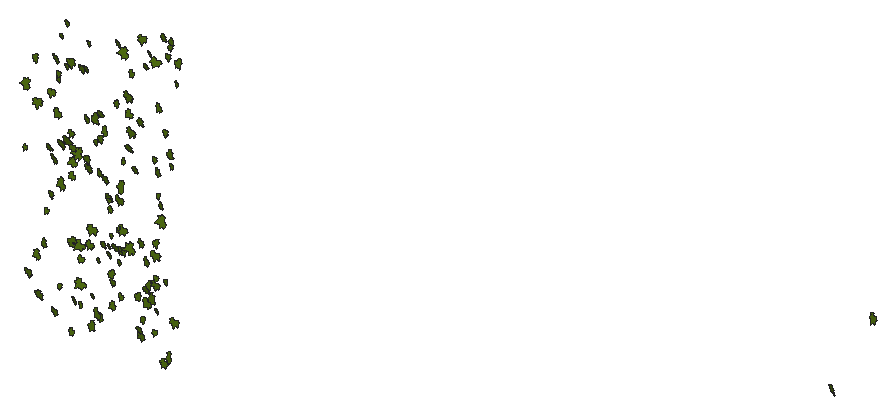
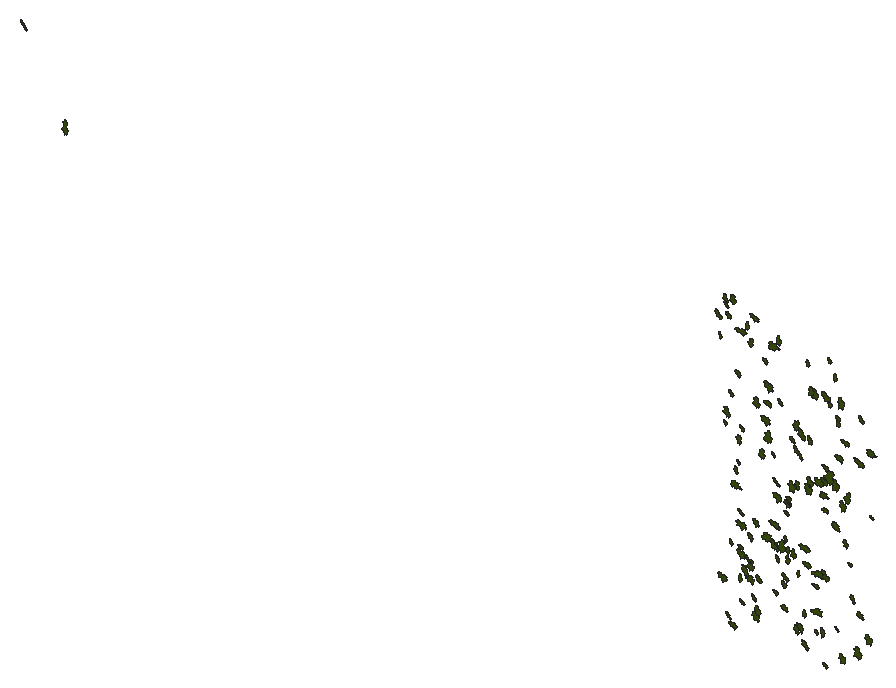
# SketchUp Ruby script. Lengths in inches.
U = 1.inch
M = Sketchup.active_model
def pt(a) = Geom::Point3d.new(a.map { |v| v * U })
def face(e, loops, mat)
  f = e.add_face(loops[0].map { |a| pt(a) })
  loops[1..].each { |l| e.add_face(l.map { |a| pt(a) }).erase! }
  f.material = f.back_material = mat if mat
  f
end
# faces: each face lists its corners as indices into pts; further lists are holes
def faces(e, pts, list, mat = nil) = list.each { |f| face(e, (f[0].is_a?(Array) ? f : [f]).map { |l| l.map { |i| pts[i] } }, mat) }
# xy, xz, yz: faces in a plane at the given z, y or x. An outline is a flat list of corners, or four numbers for a rectangle; further outlines are holes
def ring(l) = l.size == 4 ? [[l[0], l[1]], [l[2], l[1]], [l[2], l[3]], [l[0], l[3]]] : l.each_slice(2).to_a
def flat(e, list, mat, &to3) = list.each { |f| face(e, (f[0].is_a?(Array) ? f : [f]).map { |l| ring(l).map { |u, v| to3.(u, v) } }, mat) }
def xy(e, z, list, mat = nil) = flat(e, list, mat) { |x, y| [x, y, z] }
def xz(e, y, list, mat = nil) = flat(e, list, mat) { |x, z| [x, y, z] }
def yz(e, x, list, mat = nil) = flat(e, list, mat) { |y, z| [x, y, z] }
def lines(e, pts, list) = list.each { |a, b| e.add_line(pt(pts[a]), pt(pts[b])) }
# prism: a flat outline (further loops are holes) pulled along v
def prism(e, loops, v, mat = nil)
  f = face(e, loops, mat); d = Geom::Vector3d.new(v.map { |x| x * U })
  f.pushpull(f.normal.samedirection?(d) ? d.length : -d.length)
end
def box(e, o, s, mat = nil) = prism(e, [[o, [o[0] + s[0], o[1], o[2]], [o[0] + s[0], o[1] + s[1], o[2]], [o[0], o[1] + s[1], o[2]]]], [0, 0, s[2]], mat)
def at(x, y, z, deg = 0) = Geom::Transformation.translation(pt([x, y, z])) * Geom::Transformation.rotation(ORIGIN, Z_AXIS, deg.degrees)
def axes(o, x, y, z) = Geom::Transformation.new([*x, 0, *y, 0, *z, 0, *pt(o).to_a, 1])
def part(name) = M.definitions.add(name)
# library, detail: a bought-in or finely detailed component or shape, given as its bounding box
def library(name, o, s) = part(name).tap { |d| box(d.entities, o, s) }
def detail(e, o, s) = box(e.add_group.entities, o, s)
def put(e, d, t, mat = nil) = e.add_instance(d, t).tap { |i| i.material = mat if mat }
def group(e, t, mat = nil) = e.add_group.tap { |g| g.transformation = t; g.material = mat if mat }.entities
root = M.entities
M.materials.add("[Vegetation Blur 03]").color = [83, 114, 18]
c1 = part("ivy")
xy(c1.entities,0,[[0.782,0,0.786,0,0.787,0.005,0.789,0.009,0.821,0.072,0.875,0.147,1.001,0.272,1.073,0.331,1.137,0.363,1.178,0.379,1.223,0.384,1.272,0.383,1.311,0.374,1.36,0.355,1.399,0.334,1.491,0.285,1.541,0.244,1.583,0.199,1.617,0.15,1.64,0.128,1.662,0.115,1.717,0.105,1.745,0.093,1.784,0.054,1.819,0.057,1.854,0.064,1.882,0.075,1.896,0.074,1.91,0.071,1.937,0.063,1.964,0.053,1.99,0.038,2.016,0.015,2.034,0.002,2.04,0,2.038,0.003,2.036,0.007,2.033,0.038,2.036,0.068,2.045,0.1,2.055,0.116,2.064,0.123,2.077,0.129,2.088,0.129,2.106,0.132,2.118,0.13,2.179,0.132,2.207,0.133,2.225,0.133,2.242,0.138,2.22,0.162,2.207,0.186,2.206,0.213,2.212,0.236,2.228,0.262,2.247,0.274,2.298,0.283,2.355,0.294,2.37,0.296,2.376,0.295,2.377,0.3,2.377,0.303,2.385,0.329,2.411,0.37,2.426,0.392,2.449,0.407,2.511,0.426,2.561,0.444,2.619,0.466,2.589,0.469,2.561,0.476,2.501,0.5,2.449,0.516,2.424,0.523,2.401,0.535,2.377,0.556,2.372,0.568,2.36,0.575,2.268,0.586,2.225,0.592,2.207,0.599,2.194,0.61,2.143,0.65,2.13,0.664,2.122,0.682,2.123,0.7,2.13,0.719,2.148,0.75,2.17,0.781,2.195,0.807,2.221,0.828,2.284,0.874,2.291,0.88,2.288,0.887,2.276,0.9,2.267,0.916,2.265,0.933,2.273,0.967,2.292,1.002,2.313,1.03,2.334,1.054,2.348,1.067,2.358,1.074,2.363,1.076,2.362,1.081,2.35,1.094,2.347,1.11,2.35,1.143,2.359,1.18,2.385,1.254,2.415,1.324,2.448,1.393,2.45,1.4,2.446,1.398,2.44,1.394,2.427,1.383,2.402,1.36,2.376,1.339,2.345,1.324,2.305,1.309,2.282,1.303,2.273,1.306,2.245,1.294,2.212,1.287,2.187,1.291,2.163,1.301,2.142,1.316,2.134,1.327,2.124,1.325,2.09,1.292,2.053,1.259,2.014,1.234,1.973,1.215,1.954,1.21,1.931,1.208,1.909,1.212,1.893,1.22,1.879,1.233,1.872,1.248,1.867,1.281,1.864,1.319,1.821,1.258,1.773,1.197,1.726,1.141,1.698,1.121,1.679,1.116,1.666,1.117,1.647,1.122,1.632,1.129,1.62,1.141,1.617,1.154,1.617,1.219,1.621,1.254,1.623,1.268,1.623,1.281,1.618,1.314,1.606,1.346,1.603,1.375,1.607,1.403,1.603,1.467,1.599,1.499,1.605,1.525,1.614,1.552,1.629,1.577,1.635,1.589,1.629,1.587,1.618,1.582,1.596,1.566,1.581,1.556,1.568,1.552,1.557,1.55,1.545,1.553,1.531,1.562,1.522,1.572,1.504,1.591,1.486,1.611,1.474,1.631,1.457,1.666,1.455,1.684,1.457,1.698,1.452,1.715,1.444,1.728,1.424,1.754,1.419,1.772,1.423,1.786,1.434,1.819,1.444,1.848,1.446,1.855,1.44,1.861,1.43,1.867,1.386,1.904,1.349,1.948,1.326,1.973,1.31,1.995,1.288,2.048,1.284,2.153,1.287,2.254,1.284,2.255,1.282,2.253,1.278,2.247,1.274,2.237,1.266,2.216,1.226,2.125,1.208,2.076,1.184,2.033,1.155,1.984,1.135,1.942,1.111,1.899,1.083,1.861,1.053,1.85,1.059,1.83,1.061,1.809,1.056,1.79,1.049,1.767,1.04,1.749,1.018,1.733,0.994,1.726,0.942,1.734,0.95,1.6875,0.944,1.645,0.932,1.608,0.911,1.585,0.881,1.58,0.854,1.582,0.828,1.588,0.785,1.618,0.773,1.625,0.775,1.614,0.779,1.598,0.796,1.502,0.818,1.402,0.861,1.283,0.882,1.224,0.894,1.174,0.892,1.148,0.886,1.123,0.881,1.107,0.872,1.099,0.849,1.094,0.818,1.092,0.789,1.098,0.762,1.107,0.753,1.113,0.721,1.139,0.698,1.163,0.678,1.194,0.665,1.224,0.628,1.28,0.612,1.312,0.606,1.327,0.606,1.314,0.599,1.282,0.594,1.267,0.581,1.256,0.544,1.245,0.512,1.244,0.473,1.249,0.444,1.256,0.382,1.288,0.339,1.306,0.324,1.316,0.317,1.324,0.309,1.326,0.27,1.314,0.227,1.313,0.185,1.3125,0.152,1.317,0.122,1.328,0.092,1.345,0.073,1.353,0.079,1.338,0.092,1.308,0.117,1.249,0.13,1.215,0.139,1.164,0.147,1.148,0.157,1.136,0.163,1.122,0.174,1.086,0.177,1.067,0.182,1.054,0.186,1.043,0.191,1.038,0.211,1.028,0.237,1.005,0.25,0.974,0.253,0.96,0.25,0.944,0.242,0.914,0.243,0.906,0.249,0.902,0.26,0.894,0.289,0.88,0.307,0.873,0.322,0.862,0.364,0.799,0.403,0.738,0.431,0.709,0.439,0.691,0.441,0.678,0.4375,0.66,0.428,0.645,0.394,0.623,0.303,0.594,0.255,0.581,0.214,0.577,0.179,0.573,0.173,0.568,0.175,0.561,0.167,0.55,0.141,0.523,0.113,0.503,0.077,0.49,0.045,0.486,0.026,0.485,0.019,0.486,0.011,0.483,0,0.471,0.014,0.467,0.044,0.455,0.058,0.447,0.07,0.438,0.097,0.411,0.125,0.394,0.158,0.377,0.174,0.366,0.182,0.359,0.185,0.361,0.242,0.331,0.253,0.316,0.258,0.303,0.262,0.283,0.274,0.278,0.308,0.274,0.341,0.252,0.366,0.226,0.366,0.222,0.37,0.22,0.38,0.221,0.395,0.221,0.425,0.216,0.45,0.207,0.465,0.192,0.473,0.178,0.484,0.15,0.489,0.116,0.483,0.089,0.468,0.058,0.45,0.035,0.435,0.018,0.429,0.011,0.434,0.012,0.438,0.014,0.469,0.019,0.542,0.016,0.581,0.015,0.612,0.027,0.68,0.055,0.696,0.057,0.712,0.052,0.73,0.045,0.741,0.036,0.766,0.014]])
put(root,c1,axes([24.02,173.2,118.26],[0.59751,-0.1415,-0.08723],[-0.11552,-0.16395,-0.48523],[-0.05298,-1.23827,0.07421]),"[Vegetation Blur 03]")
put(root,c1,axes([30.52,173.2,121.6875],[0.30037,-0.23448,-0.48095],[-0.59958,-0.05449,-0.24524],[-0.02777,-1.36002,0.09275]),"[Vegetation Blur 03]")
put(root,c1,axes([14.2,173.2,137.15],[0.5598,-0.34639,0.09978],[0.13771,0.07562,-0.47332],[-0.15594,-1.17668,-0.05979]),"[Vegetation Blur 03]")
put(root,c1,axes([11.29,173.2,135.72],[0.34108,-0.07651,0.26436],[0.30846,-0.23678,-0.27587],[-0.10562,-0.93855,0.04805]),"[Vegetation Blur 03]")
put(root,c1,axes([32.13,173.2,139.74],[0.30667,-0.21087,0.08542],[0.09735,-0.07998,-0.26385],[-0.10945,-0.662,0.00467]),"[Vegetation Blur 03]")
put(root,c1,axes([22.87,173.2,114.92],[0.32867,-0.28906,0.36046],[0.45664,0.0115,-0.27589],[-0.07923,-1.13284,-0.09478]),"[Vegetation Blur 03]")
put(root,c1,axes([31.43,173.2,104.15],[0.33567,-0.36714,-0.32626],[-0.40941,0.10373,-0.29893],[-0.15499,-1.06915,0.08303]),"[Vegetation Blur 03]")
put(root,c1,axes([23.38,173.2,142.01],[0.40968,-0.27629,0.16507],[0.21084,0.00024,-0.34848],[-0.12034,-0.94019,-0.0486]),"[Vegetation Blur 03]")
put(root,c1,axes([13.45,173.2,124.49],[0.13916,-0.21976,0.37305],[0.46529,-0.06512,-0.12164],[-0.06205,-0.98109,-0.07549]),"[Vegetation Blur 03]")
put(root,c1,axes([30.39,173.2,132.73],[0.36627,-0.13941,0.12421],[0.13945,-0.15724,-0.30166],[-0.09113,-0.8009,0.0376]),"[Vegetation Blur 03]")
put(root,c1,axes([16.95,173.2,102.27],[0.36884,-0.18268,-0.08765],[-0.12074,-0.10682,-0.30338],[-0.06956,-0.78327,0.06182]),"[Vegetation Blur 03]")
put(root,c1,axes([15.09,173.2,107.24],[0.27201,-0.08351,0.1346],[0.14493,-0.22002,-0.21655],[-0.08857,-0.61651,0.05905]),"[Vegetation Blur 03]")
put(root,c1,axes([27.82,173.2,111.51],[0.22572,0.02556,0.3673],[0.42622,-0.34586,-0.17068],[-0.14503,-0.97663,0.07006]),"[Vegetation Blur 03]")
put(root,c1,axes([11.59,173.2,105.01],[0.44693,-0.21309,0.34937],[0.42945,-0.06761,-0.37241],[-0.09772,-1.27172,-0.03874]),"[Vegetation Blur 03]")
put(root,c1,axes([29.58,173.2,136.08],[0.46163,-0.2581,-0.13642],[-0.17424,-0.01487,-0.3883],[-0.11538,-1.01019,0.04057]),"[Vegetation Blur 03]")
put(root,c1,axes([29.79,173.2,122.5625],[0.11578,-0.07742,0.31422],[0.36947,-0.22297,-0.09932],[-0.11465,-0.79672,-0.00274]),"[Vegetation Blur 03]")
put(root,c1,axes([20.81,173.2,128.5],[0.35673,-0.12377,0.22075],[0.25958,-0.16822,-0.29423],[-0.09696,-0.90576,0.02448]),"[Vegetation Blur 03]")
put(root,c1,axes([11.39,173.2,130.33],[0.60257,-0.08021,0.1387],[0.16152,-0.21723,-0.48713],[-0.06569,-1.26991,0.07457]),"[Vegetation Blur 03]")
put(root,c1,axes([21.97,173.2,120.94],[0.20255,-0.18759,0.41357],[0.50926,-0.09194,-0.17269],[-0.07578,-1.11921,-0.05513]),"[Vegetation Blur 03]")
put(root,c1,axes([16.01,173.2,126.02],[0.0827,-0.23642,0.52033],[0.64705,-0.03418,-0.07095],[-0.03151,-1.3225,-0.09118]),"[Vegetation Blur 03]")
put(root,c1,axes([24.58,173.2,127.12],[0.30532,-0.22387,-0.07925],[-0.10993,-0.04866,-0.26046],[-0.09582,-0.65751,0.04626]),"[Vegetation Blur 03]")
put(root,c1,axes([23.22,173.2,133.91],[0.28926,-0.09005,0.2261],[0.2622,-0.20395,-0.23621],[-0.09958,-0.79857,0.03483]),"[Vegetation Blur 03]")
put(root,c1,axes([22.54,173.2,120.12],[0.34373,-0.18323,-0.04475],[-0.06771,-0.09451,-0.28552],[-0.07969,-0.71,0.04955]),"[Vegetation Blur 03]")
put(root,c1,axes([13.64,173.2,118.84],[0.37427,-0.16845,0.18276],[0.21743,-0.11081,-0.31265],[-0.09784,-0.89065,0.00433]),"[Vegetation Blur 03]")
put(root,c1,axes([27.43,173.2,110.87],[0.2552,-0.21443,0.36363],[0.45118,-0.05704,-0.2162],[-0.07626,-1.05507,-0.06222]),"[Vegetation Blur 03]")
put(root,c1,axes([23.73,173.2,113.51],[0.3306,-0.20851,0.08999],[0.10594,-0.063,-0.2822],[-0.10584,-0.71438,-0.00138]),"[Vegetation Blur 03]")
put(root,c1,axes([18.64,173.2,126.18],[0.08303,-0.1967,-0.5076],[-0.62878,-0.07669,-0.06383],[0.02474,-1.28895,0.08126]),"[Vegetation Blur 03]")
put(root,c1,axes([18.94,173.2,130.79],[0.45964,-0.254,0.03008],[0.03689,-0.00973,-0.3884],[-0.12342,-0.94883,-0.00407]),"[Vegetation Blur 03]")
put(root,c1,axes([20.56,173.2,106.22],[0.52518,-0.29878,-0.23016],[-0.2856,0.04291,-0.44284],[-0.13799,-1.22592,0.0406]),"[Vegetation Blur 03]")
put(root,c1,axes([16.22,173.2,137.1],[0.56013,-0.13091,0.22183],[0.26451,-0.15182,-0.45897],[-0.08921,-1.27215,0.03195]),"[Vegetation Blur 03]")
put(root,c1,axes([30.02,173.2,144.75],[0.24867,-0.15858,0.33537],[0.40835,-0.11898,-0.21053],[-0.08971,-0.98119,-0.02867]),"[Vegetation Blur 03]")
put(root,c1,axes([22.29,173.2,114.86],[0.1642,-0.18374,0.20113],[0.24769,-0.08699,-0.14719],[-0.08574,-0.60314,-0.04004]),"[Vegetation Blur 03]")
put(root,c1,axes([28.11,173.2,142.38],[0.3403,-0.29163,0.09942],[0.13762,0.03874,-0.29588],[-0.12643,-0.74278,-0.05447]),"[Vegetation Blur 03]")
put(root,c1,axes([27.04,173.2,107.01],[0.30019,-0.07683,0.21744],[0.25164,-0.21034,-0.24309],[-0.09515,-0.7987,0.0431]),"[Vegetation Blur 03]")
put(root,c1,axes([17.96,173.2,136.88],[0.47833,-0.24749,0.17674],[0.22101,-0.01127,-0.40089],[-0.11188,-1.08043,-0.0363]),"[Vegetation Blur 03]")
put(root,c1,axes([30.26,173.2,102.99],[0.48428,-0.17048,-0.13656],[-0.17611,-0.0992,-0.39652],[-0.06201,-1.04969,0.05965]),"[Vegetation Blur 03]")
put(root,c1,axes([28.81,173.2,128.67],[0.3385,-0.12078,0.12895],[0.14584,-0.15588,-0.27795],[-0.08451,-0.75275,0.03687]),"[Vegetation Blur 03]")
put(root,c1,axes([19.52,173.2,116.72],[0.62885,-0.10059,-0.07918],[-0.103,-0.17922,-0.50906],[-0.03454,-1.29703,0.07648]),"[Vegetation Blur 03]")
put(root,c1,axes([24,173.2,114.98],[0.40007,-0.13518,0.27607],[0.33165,-0.13835,-0.33079],[-0.0935,-1.06919,0.0079]),"[Vegetation Blur 03]")
put(root,c1,axes([23.77,173.2,114.53],[0.13511,-0.04438,0.35866],[0.42367,-0.24214,-0.11102],[-0.11873,-0.91459,0.01199]),"[Vegetation Blur 03]")
put(root,c1,axes([25.83,173.2,126.07],[0.25746,-0.20708,0.31713],[0.39391,-0.05224,-0.21837],[-0.07715,-0.95777,-0.05666]),"[Vegetation Blur 03]")
put(root,c1,axes([14.8,173.2,130.3],[0.50454,-0.20666,-0.19788],[-0.2502,-0.0525,-0.4163],[-0.0792,-1.15072,0.05453]),"[Vegetation Blur 03]")
put(root,c1,axes([26.52,173.2,132.5],[0.30631,-0.15054,0.36025],[0.43855,-0.11732,-0.25607],[-0.08874,-1.09937,-0.022]),"[Vegetation Blur 03]")
put(root,c1,axes([26.79,173.2,143.9375],[0.54024,-0.08088,0.09089],[0.10321,-0.19815,-0.43637],[-0.05739,-1.11765,0.07079]),"[Vegetation Blur 03]")
put(root,c1,axes([14.9,173.2,126.11],[0.57292,-0.29787,0.17247],[0.22282,0.05394,-0.47834],[-0.12636,-1.25544,-0.06147]),"[Vegetation Blur 03]")
put(root,c1,axes([28.14,173.2,109.62],[0.16056,0.04012,0.53459],[0.63688,-0.33645,-0.12344],[-0.15436,-1.34643,0.04677]),"[Vegetation Blur 03]")
put(root,c1,axes([26.81,173.2,117.41],[0.49502,-0.2424,-0.04719],[-0.06027,-0.00753,-0.41504],[-0.11656,-1.02555,0.0142]),"[Vegetation Blur 03]")
put(root,c1,axes([24.73,173.2,135.95],[0.66254,-0.24066,-0.04091],[-0.05165,-0.00895,-0.54898],[-0.11628,-1.36725,0.01079]),"[Vegetation Blur 03]")
put(root,c1,axes([22.05,173.2,121.33],[0.43109,-0.16307,0.09857],[0.11374,-0.09903,-0.3571],[-0.08905,-0.91592,0.02106]),"[Vegetation Blur 03]")
put(root,c1,axes([31.18,173.2,144.58],[0.22749,-0.09368,0.31124],[0.37139,-0.17878,-0.18927],[-0.09787,-0.89612,0.00522]),"[Vegetation Blur 03]")
put(root,c1,axes([19.43,173.2,114.61],[0.48596,-0.138,-0.11802],[-0.15256,-0.12597,-0.39525],[-0.04619,-1.03571,0.0638]),"[Vegetation Blur 03]")
put(root,c1,axes([25.83,173.2,116.5],[0.32603,-0.13943,-0.47145],[-0.58131,-0.12239,-0.26207],[0.01889,-1.35947,0.07195]),"[Vegetation Blur 03]")
put(root,c1,axes([29.16,173.2,108.93],[0.26661,-0.22568,0.1584],[0.20153,-0.02212,-0.2309],[-0.09528,-0.67823,-0.04518]),"[Vegetation Blur 03]")
put(root,c1,axes([20.31,173.2,127.85],[0.25768,-0.12141,0.16925],[0.19637,-0.14245,-0.21521],[-0.08903,-0.66558,0.01519]),"[Vegetation Blur 03]")
put(root,c1,axes([20.82,173.2,123.65],[0.09017,-0.06413,0.35822],[0.42718,-0.20848,-0.07749],[-0.10559,-0.89821,-0.00759]),"[Vegetation Blur 03]")
put(root,c1,axes([24.71,173.2,124.09],[0.21833,-0.37386,-0.44692],[-0.55988,0.15366,-0.2024],[-0.13932,-1.20335,0.113]),"[Vegetation Blur 03]")
put(root,c1,axes([16.6875,173.2,128.09],[0.442,-0.16404,-0.03453],[-0.05057,-0.08968,-0.36412],[-0.07475,-0.90929,0.04214]),"[Vegetation Blur 03]")
put(root,c1,axes([17.91,173.2,114.2],[0.52837,-0.04737,-0.26503],[-0.32337,-0.22367,-0.42312],[0.03764,-1.25647,0.08531]),"[Vegetation Blur 03]")
put(root,c1,axes([24.75,173.2,128.62],[0.38193,-0.25872,0.35613],[0.44798,0.02235,-0.31745],[-0.07443,-1.19311,-0.08317]),"[Vegetation Blur 03]")
put(root,c1,axes([30.46,173.2,113.14],[0.25479,-0.12423,0.18023],[0.21133,-0.13383,-0.2135],[-0.08804,-0.68079,0.00908]),"[Vegetation Blur 03]")
put(root,c1,axes([30.7,173.2,142.8],[0.3823,-0.12513,0.1329],[0.15394,-0.13225,-0.31454],[-0.08072,-0.8448,0.02956]),"[Vegetation Blur 03]")
put(root,c1,axes([25.34,173.2,133.8],[0.41213,-0.1677,-0.21359],[-0.27008,-0.08234,-0.33694],[-0.04682,-1.00125,0.06348]),"[Vegetation Blur 03]")
put(root,c1,axes([10.11,173.2,107.66],[0.54065,-0.21536,0.14176],[0.17436,-0.02611,-0.44914],[-0.10356,-1.16826,-0.01609]),"[Vegetation Blur 03]")
put(root,c1,axes([23.02,173.2,107.9],[0.35443,-0.19304,-0.2419],[-0.30587,-0.0509,-0.29211],[-0.05567,-0.94941,0.06485]),"[Vegetation Blur 03]")
put(root,c1,axes([29.29,173.2,126.59],[0.06006,-0.04189,0.40073],[0.47866,-0.22553,-0.0515],[-0.11129,-0.99263,-0.00521]),"[Vegetation Blur 03]")
put(root,c1,axes([31.97,173.2,142.17],[0.38148,-0.02964,0.33346],[0.3977,-0.23961,-0.3064],[-0.09475,-1.12505,0.05647]),"[Vegetation Blur 03]")
put(root,c1,axes([19.8,173.2,130.52],[0.31957,-0.02324,0.46113],[0.55443,-0.24575,-0.25788],[-0.10943,-1.31297,0.04011]),"[Vegetation Blur 03]")
put(root,c1,axes([25.14,173.2,141.66],[0.17867,-0.14742,-0.47769],[-0.58909,-0.10072,-0.14187],[0.02629,-1.25528,0.06748]),"[Vegetation Blur 03]")
put(root,c1,axes([21.33,173.2,123.72],[0.52923,-0.27231,0.14829],[0.19148,0.04522,-0.44212],[-0.11773,-1.15056,-0.05247]),"[Vegetation Blur 03]")
put(root,c1,axes([18.09,173.2,109.21],[0.5099,-0.05447,-0.26558],[-0.32487,-0.20771,-0.40876],[0.03235,-1.22728,0.08097]),"[Vegetation Blur 03]")
put(root,c1,axes([19.3,173.2,140.57],[0.32682,-0.209,0.08086],[0.0994,-0.02803,-0.27901],[-0.10124,-0.70219,-0.01293]),"[Vegetation Blur 03]")
put(root,c1,axes([30.85,173.2,129.63],[0.21618,-0.06557,0.43271],[0.52184,-0.19331,-0.17826],[-0.09899,-1.16227,0.00524]),"[Vegetation Blur 03]")
put(root,c1,axes([10.08,173.2,123.76],[0.29106,-0.10296,0.03164],[0.02588,-0.14904,-0.23485],[-0.05776,-0.58557,0.05421]),"[Vegetation Blur 03]")
put(root,c1,axes([26.37,173.2,105.71],[0.48095,-0.24511,0.14889],[0.18901,0.01686,-0.4023],[-0.10837,-1.05836,-0.04089]),"[Vegetation Blur 03]")
put(root,c1,axes([27.73,173.2,115.37],[0.45232,-0.27078,-0.13351],[-0.16346,0.04761,-0.38403],[-0.13176,-0.98864,0.01808]),"[Vegetation Blur 03]")
put(root,c1,axes([31.44,173.2,128.8125],[0.32645,-0.19251,-0.02516],[-0.03795,-0.04316,-0.27603],[-0.0909,-0.67338,0.02489]),"[Vegetation Blur 03]")
put(root,c1,axes([25.65,173.2,139.04],[0.38208,-0.19358,-0.10183],[-0.13229,-0.03969,-0.31874],[-0.08317,-0.82615,0.03917]),"[Vegetation Blur 03]")
put(root,c1,axes([13.24,173.2,116.64],[0.31975,-0.13436,-0.03342],[-0.05173,-0.10756,-0.26163],[-0.05713,-0.65457,0.04985]),"[Vegetation Blur 03]")
put(root,c1,axes([15.3,173.2,139.92],[0.22551,-0.17157,0.19026],[0.23404,-0.06401,-0.19384],[-0.08079,-0.66437,-0.03046]),"[Vegetation Blur 03]")
put(root,c1,axes([29.41,173.2,123.97],[0.2323,-0.07315,0.16912],[0.19295,-0.17827,-0.18866],[-0.08352,-0.61528,0.03456]),"[Vegetation Blur 03]")
put(root,c1,axes([18.13,173.2,112.16],[0.41492,-0.08686,-0.03354],[-0.04844,-0.1605,-0.33372],[-0.03354,-0.84286,0.067]),"[Vegetation Blur 03]")
put(root,c1,axes([12.125,173.2,110.86],[0.33179,-0.22508,-0.3253],[-0.40723,0.00189,-0.27687],[-0.0707,-1.0672,0.06812]),"[Vegetation Blur 03]")
put(root,c1,axes([28.76,173.2,112.54],[0.56428,-0.16916,0.04285],[0.04868,-0.06133,-0.46503],[-0.08453,-1.16458,0.01826]),"[Vegetation Blur 03]")
put(root,c1,axes([28.8125,173.2,141.82],[0.58164,-0.02914,-0.08506],[-0.10504,-0.22356,-0.46637],[0.00547,-1.19524,0.0893]),"[Vegetation Blur 03]")
put(root,c1,axes([18.7,173.2,125.14],[0.40671,-0.14437,0.24599],[0.29835,-0.08915,-0.33679],[-0.0822,-1.03788,-0.00529]),"[Vegetation Blur 03]")
put(root,c1,axes([20.76,173.2,112.33],[0.10915,-0.09215,0.23401],[0.27778,-0.14927,-0.09555],[-0.08399,-0.61343,-0.0119]),"[Vegetation Blur 03]")
put(root,c1,axes([17.53,173.2,124.7],[0.25465,-0.11048,-0.36792],[-0.45313,-0.12762,-0.20287],[0.02807,-1.05778,0.0629]),"[Vegetation Blur 03]")
put(root,c1,axes([24.01,173.2,109.24],[0.37736,-0.14693,-0.03133],[-0.04655,-0.08489,-0.31089],[-0.06637,-0.77592,0.03994]),"[Vegetation Blur 03]")
put(root,c1,axes([20.92,173.2,131.4],[0.10455,-0.16948,0.36645],[0.45413,-0.0579,-0.09052],[-0.04648,-0.94693,-0.06005]),"[Vegetation Blur 03]")
put(root,c1,axes([28.88,173.2,106.16],[0.34421,-0.10508,0.04416],[0.04441,-0.1326,-0.28022],[-0.05969,-0.70465,0.04615]),"[Vegetation Blur 03]")
put(root,c1,axes([10.9,173.2,132.65],[0.1603,-0.20672,-0.46475],[-0.57787,-0.01388,-0.13179],[-0.02063,-1.21728,0.08043]),"[Vegetation Blur 03]")
put(root,c1,axes([18.88,173.2,124.36],[0.58972,-0.25941,0.10506],[0.13617,0.04808,-0.49046],[-0.11798,-1.24117,-0.04096]),"[Vegetation Blur 03]")
put(root,c1,axes([14.79,173.2,134.21],[0.29872,-0.15455,0.15212],[0.18312,-0.07365,-0.25129],[-0.08276,-0.72081,-0.00694]),"[Vegetation Blur 03]")
put(root,c1,axes([22,173.2,130.34],[0.30417,-0.25351,-0.27604],[-0.3464,0.04167,-0.26026],[-0.0979,-0.93513,0.06323]),"[Vegetation Blur 03]")
put(root,c1,axes([20.875,173.2,104.72],[0.09186,-0.01547,0.40746],[0.48625,-0.23456,-0.07442],[-0.11344,-1.01793,0.01096]),"[Vegetation Blur 03]")
put(root,c1,axes([31.07,173.2,143.92],[0.26564,-0.06538,0.20861],[0.24422,-0.17627,-0.21582],[-0.08188,-0.73784,0.03307]),"[Vegetation Blur 03]")
put(root,c1,axes([14.05,173.2,103.93],[0.51714,-0.23527,0.06533],[0.0842,0.02179,-0.43163],[-0.1113,-1.07662,-0.02301]),"[Vegetation Blur 03]")
put(root,c1,axes([16.72,173.2,126.17],[0.49069,-0.15556,0.05335],[0.06086,-0.06942,-0.40473],[-0.07927,-1.0163,0.01948]),"[Vegetation Blur 03]")
put(root,c1,axes([13.6,173.2,132.3125],[0.49447,-0.06651,0.04707],[0.05156,-0.17262,-0.39913],[-0.04138,-1.00977,0.06513]),"[Vegetation Blur 03]")
put(root,c1,axes([17.11,173.2,106.47],[0.46353,-0.32199,-0.04056],[-0.03174,0.12476,-0.39742],[-0.16108,-0.95117,-0.0384]),"[Vegetation Blur 03]")
put(root,c1,axes([13.97,173.2,123.97],[0.56984,-0.3114,0.00181],[0.01697,0.11385,-0.47886],[-0.15039,-1.16708,-0.04719]),"[Vegetation Blur 03]")
put(root,c1,axes([25.17,173.2,131.42],[0.63233,-0.20373,-0.05495],[-0.06893,-0.01048,-0.5222],[-0.0979,-1.30853,0.01274]),"[Vegetation Blur 03]")
put(root,c1,axes([26.57,173.2,104.97],[0.52242,-0.17809,0.13316],[0.16214,-0.04009,-0.43214],[-0.08844,-1.12553,-0.00568]),"[Vegetation Blur 03]")
put(root,c1,axes([22.57,173.2,116.32],[0.21446,-0.11197,0.17329],[0.20462,-0.11686,-0.18055],[-0.07858,-0.60992,0.00278]),"[Vegetation Blur 03]")
put(root,c1,axes([31.4,173.2,108.68],[0.62343,-0.11777,0.0104],[0.0079,-0.1089,-0.50918],[-0.0581,-1.27854,0.04241]),"[Vegetation Blur 03]")
put(root,c1,axes([27.65,173.2,139.92],[0.06833,-0.14193,0.31087],[0.38368,-0.0807,-0.06197],[-0.05132,-0.79223,-0.04938]),"[Vegetation Blur 03]")
put(root,c1,axes([22.14,173.2,113.92],[0.34195,-0.22556,0.12659],[0.16367,0.01646,-0.28987],[-0.09636,-0.7725,-0.04314]),"[Vegetation Blur 03]")
put(root,c1,axes([16.32,173.2,113.4375],[0.45366,-0.05419,0.38117],[0.46073,-0.18,-0.36926],[-0.08098,-1.3277,0.0345]),"[Vegetation Blur 03]")
put(root,c1,axes([16.02,173.2,136.34],[0.3125,-0.15896,0.12959],[0.15654,-0.05797,-0.26261],[-0.08171,-0.71898,-0.00748]),"[Vegetation Blur 03]")
put(root,c1,axes([23.55,173.2,117.52],[0.23635,-0.06465,0.19523],[0.22776,-0.16748,-0.19239],[-0.07957,-0.67142,0.02919]),"[Vegetation Blur 03]")
put(root,c1,axes([127.07,173.7,133.12],[0.43009,-0.41994,0.38446],[0.46829,-0.19735,-0.38284],[-0.21039,-1.29771,-0.06619]),"[Vegetation Blur 03]")
put(root,c1,axes([18.2,173.2,106.1],[0.29646,-0.18293,-0.03481],[-0.04858,-0.02904,-0.25162],[-0.08579,-0.61566,0.02221]),"[Vegetation Blur 03]")
put(root,c1,axes([15.69,173.2,121.4375],[0.39569,-0.25539,-0.40505],[-0.50198,0.05522,-0.33211],[-0.09868,-1.305,0.06522]),"[Vegetation Blur 03]")
put(root,c1,axes([133.33,173.7,145],[0.61554,-0.40401,-0.01131],[-0.04771,-0.21545,-0.519],[-0.19095,-1.24853,0.09322]),"[Vegetation Blur 03]")
put(root,c1,axes([27.75,173.2,110.03],[0.51915,-0.17766,-0.225],[-0.28069,-0.03421,-0.42714],[-0.06834,-1.20911,0.04515]),"[Vegetation Blur 03]")
put(root,c1,axes([19.79,173.2,107.625],[0.27556,-0.19726,0.13683],[0.17351,-0.01114,-0.23526],[-0.08482,-0.66366,-0.03672]),"[Vegetation Blur 03]")
put(root,c1,axes([28.81,173.2,117.47],[0.29882,0.02623,0.28715],[0.33985,-0.26962,-0.23169],[-0.09199,-0.91085,0.07685]),"[Vegetation Blur 03]")
put(root,c1,axes([22.31,173.2,111.31],[0.35031,-0.0224,0.27157],[0.32357,-0.21117,-0.28075],[-0.0784,-0.97156,0.05476]),"[Vegetation Blur 03]")
put(root,c1,axes([16.1,173.2,142.1],[0.3345,-0.16348,0.07359],[0.08724,-0.0471,-0.28058],[-0.08265,-0.71135,0.00167]),"[Vegetation Blur 03]")
put(root,c1,axes([18.66,173.2,137.0625],[0.39765,-0.2594,0.13842],[0.18466,0.06494,-0.33421],[-0.10274,-0.88724,-0.06493]),"[Vegetation Blur 03]")
put(root,c1,axes([22.63,173.2,110.65],[0.43055,-0.17357,0.04955],[0.0586,-0.03425,-0.35804],[-0.08583,-0.8941,0.0041]),"[Vegetation Blur 03]")
put(root,c1,axes([19.35,173.2,103.21],[0.24806,0.03915,0.43187],[0.51673,-0.28046,-0.19369],[-0.11561,-1.16947,0.06091]),"[Vegetation Blur 03]")
put(root,c1,axes([12.68,173.2,111.54],[0.07106,0.03212,0.39333],[0.4647,-0.27217,-0.05243],[-0.12873,-0.96482,0.02788]),"[Vegetation Blur 03]")
put(root,c1,axes([28.6,173.2,116.47],[0.64834,-0.11558,0.00243],[-0.00125,-0.10055,-0.52962],[-0.05623,-1.33037,0.03982]),"[Vegetation Blur 03]")
put(root,c1,axes([21.18,173.2,114.79],[0.32691,-0.16543,0.24576],[0.30294,-0.04245,-0.2729],[-0.07327,-0.91364,-0.03182]),"[Vegetation Blur 03]")
put(root,c1,axes([23.48,173.2,121.91],[0.59559,-0.20487,-0.02237],[-0.02751,0.00349,-0.49282],[-0.09953,-1.2269,0.00233]),"[Vegetation Blur 03]")
put(root,c1,axes([26.21,173.2,109.6875],[0.31135,-0.03304,0.2876],[0.34314,-0.19604,-0.25097],[-0.08184,-0.94759,0.04189]),"[Vegetation Blur 03]")
put(root,c1,axes([17.14,173.2,122.7],[0.28967,-0.12811,-0.2275],[-0.2852,-0.08534,-0.23432],[-0.01552,-0.82284,0.05972]),"[Vegetation Blur 03]")
put(root,c1,axes([14.84,173.2,135.01],[0.33002,-0.10362,0.05882],[0.06392,-0.11285,-0.27012],[-0.06037,-0.68589,0.03556]),"[Vegetation Blur 03]")
put(root,c1,axes([29.07,173.2,113.28],[0.33589,-0.10606,0.03492],[0.03467,-0.10992,-0.27466],[-0.05731,-0.68805,0.03849]),"[Vegetation Blur 03]")
